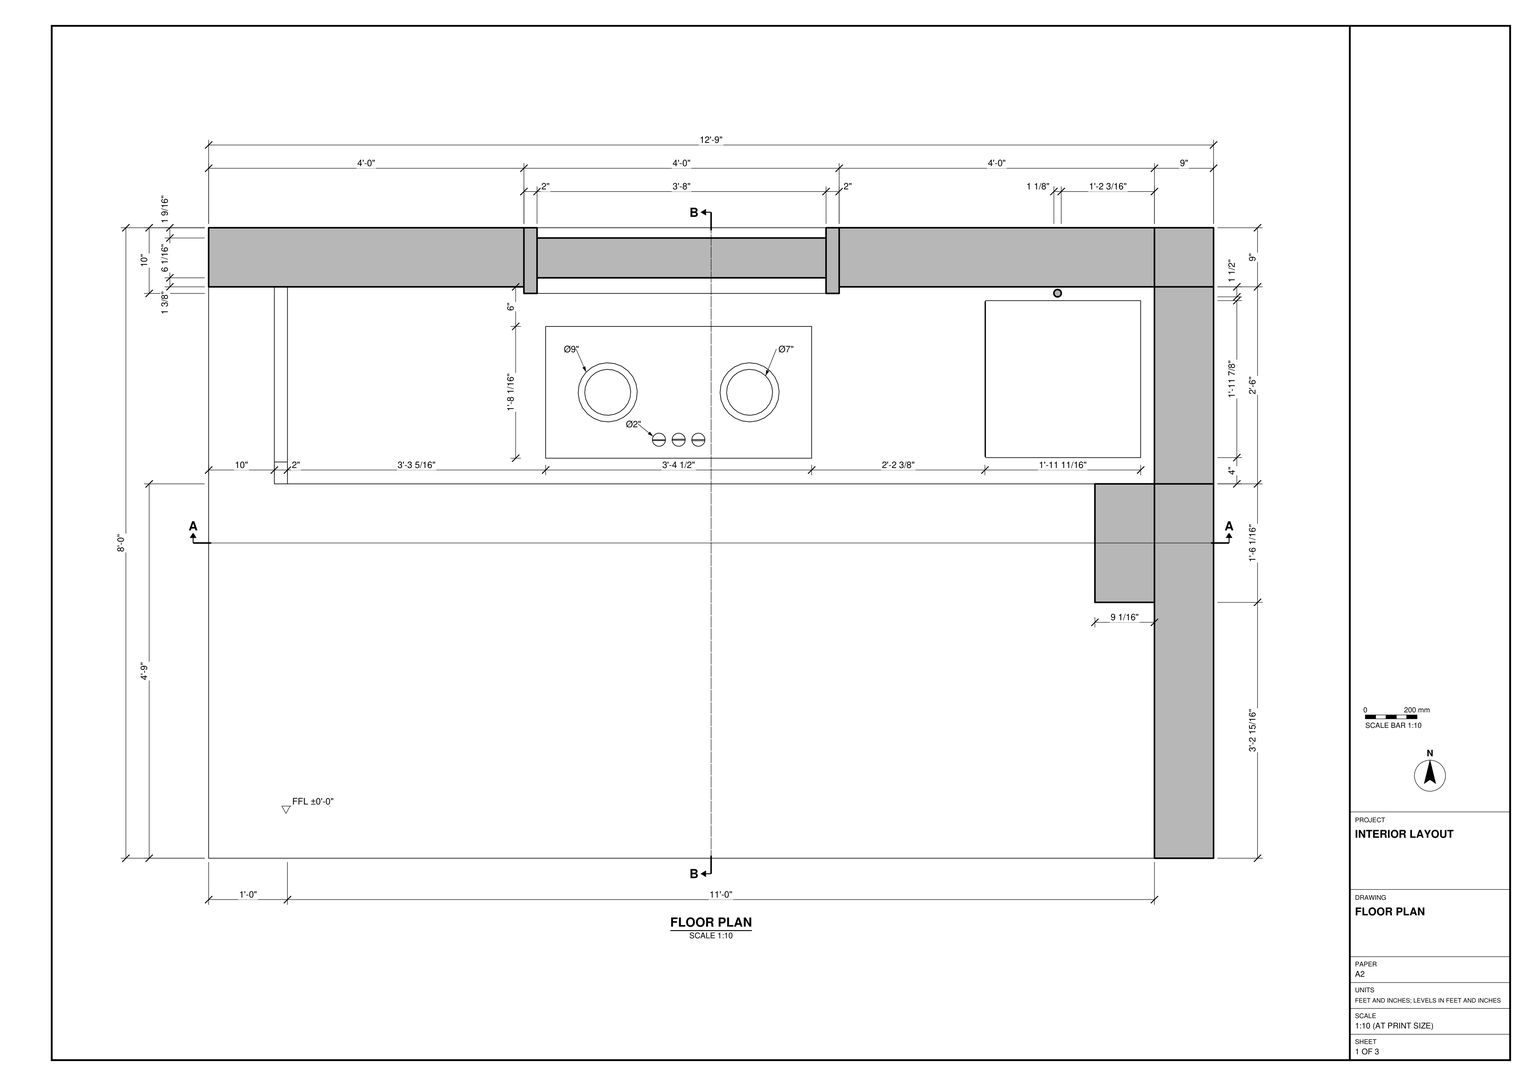
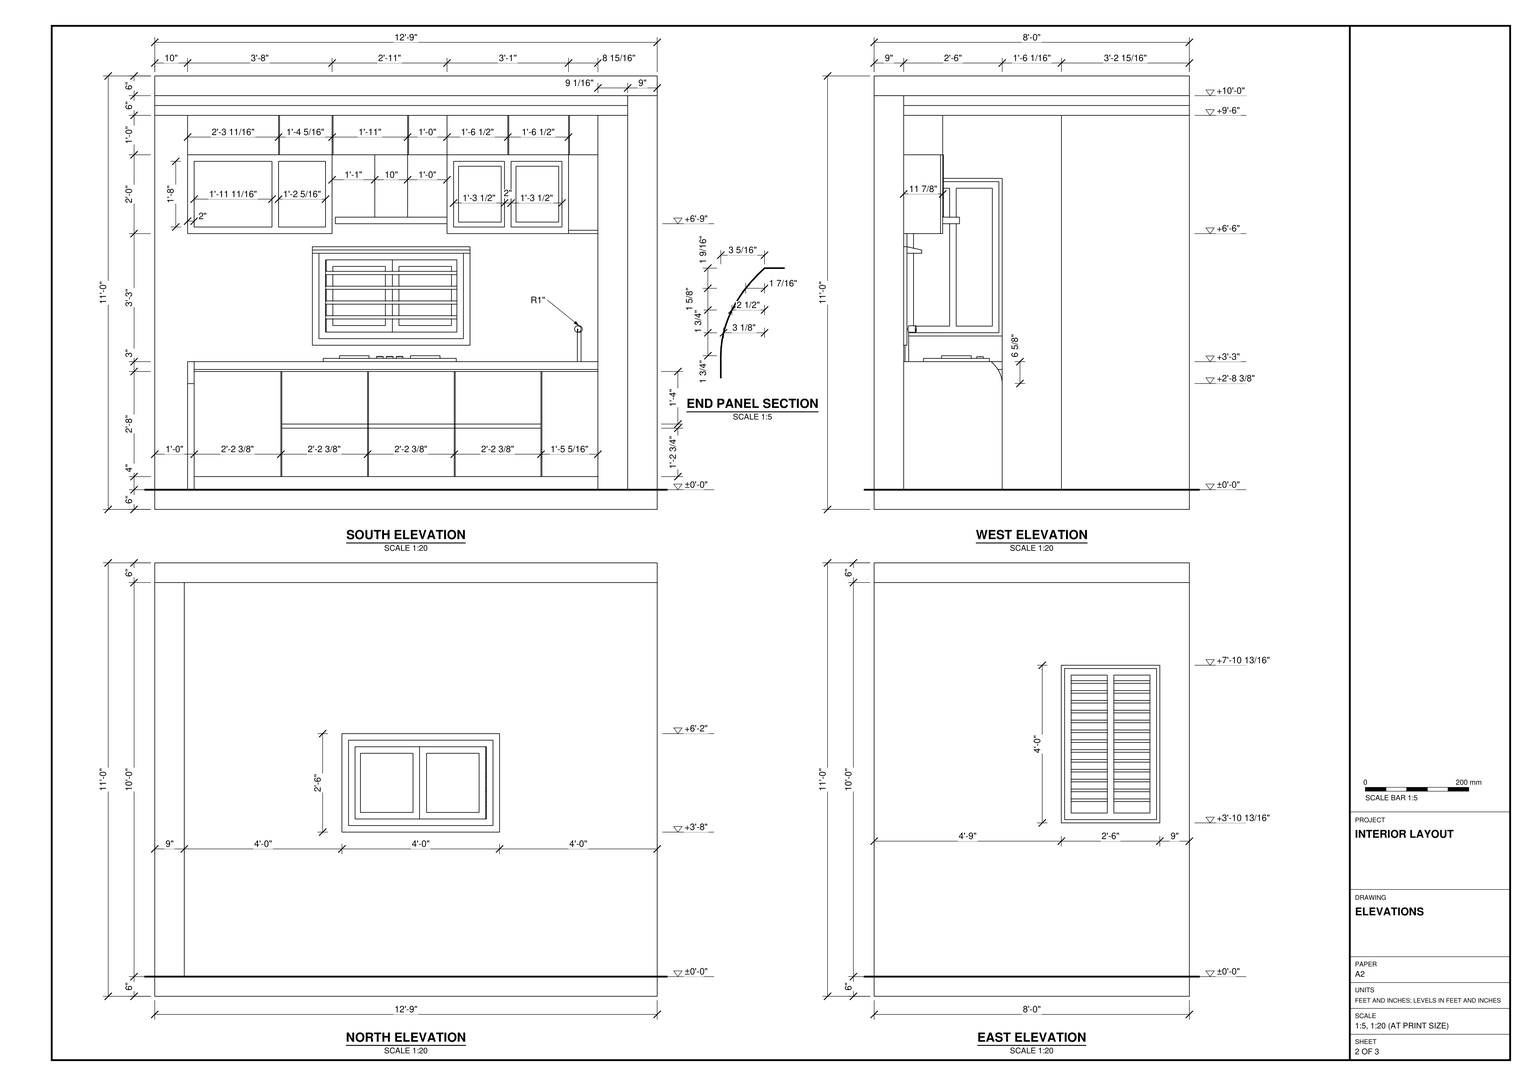
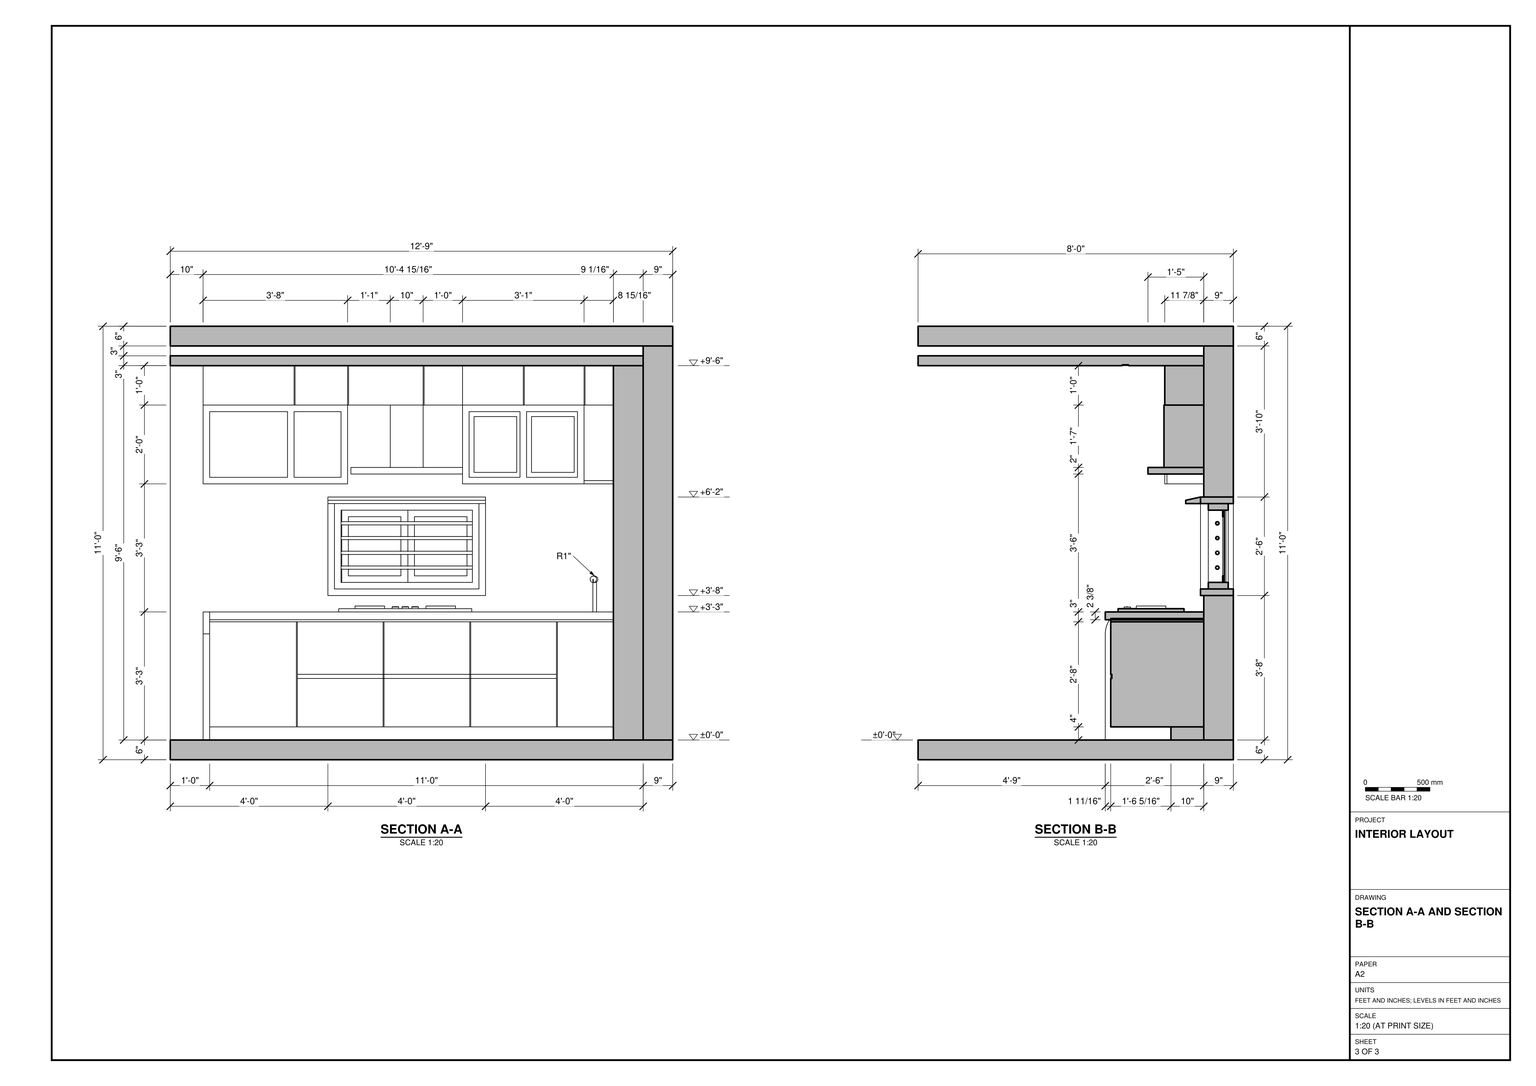
Build the kitchen interior in SketchUp from the plan, elevations and sections in task_files/diagram_01.pdf. Work in feet and inches. The overall model is 12'-9" wide, 8'-0" deep and 11'-0" high, with the finished floor at ±0'-0". Model the floor slab, the 9" thick back and right-hand walls, and the overhead slab. Leave the other two sides open as drawn. Use the sections to set the ceiling below the overhead slab and the elevations to place the two framed windows at their different sill heights.

Build the straight counter run against the back wall. Set the worktop at 3'-3" above the finished floor, with the cooktop beneath the wide window and the sink and tap at the right-hand end. Follow the south elevation for the base cabinet divisions and recessed plinth, and use the end panel section for the curved profile. Match the widths and heights of the upper cabinets and the shelf between the framed cabinet fronts. Decor, appliances and loose items may be any suitable library components.

Keep the walls, slabs, ceiling and each furniture or joinery piece in separate groups or components, and use components for repeated parts. Save one SketchUp model as output_files/kitchen_corner_and_its_built_in_cabinetry.skp.

# SketchUp Ruby script. Lengths in inches.
U = 1.inch
M = Sketchup.active_model
def pt(a) = Geom::Point3d.new(a.map { |v| v * U })
def face(e, loops, mat)
  f = e.add_face(loops[0].map { |a| pt(a) })
  loops[1..].each { |l| e.add_face(l.map { |a| pt(a) }).erase! }
  f.material = f.back_material = mat if mat
  f
end
# faces: each face lists its corners as indices into pts; further lists are holes
def faces(e, pts, list, mat = nil) = list.each { |f| face(e, (f[0].is_a?(Array) ? f : [f]).map { |l| l.map { |i| pts[i] } }, mat) }
# xy, xz, yz: faces in a plane at the given z, y or x. An outline is a flat list of corners, or four numbers for a rectangle; further outlines are holes
def ring(l) = l.size == 4 ? [[l[0], l[1]], [l[2], l[1]], [l[2], l[3]], [l[0], l[3]]] : l.each_slice(2).to_a
def flat(e, list, mat, &to3) = list.each { |f| face(e, (f[0].is_a?(Array) ? f : [f]).map { |l| ring(l).map { |u, v| to3.(u, v) } }, mat) }
def xy(e, z, list, mat = nil) = flat(e, list, mat) { |x, y| [x, y, z] }
def xz(e, y, list, mat = nil) = flat(e, list, mat) { |x, z| [x, y, z] }
def yz(e, x, list, mat = nil) = flat(e, list, mat) { |y, z| [x, y, z] }
def lines(e, pts, list) = list.each { |a, b| e.add_line(pt(pts[a]), pt(pts[b])) }
# prism: a flat outline (further loops are holes) pulled along v
def prism(e, loops, v, mat = nil)
  f = face(e, loops, mat); d = Geom::Vector3d.new(v.map { |x| x * U })
  f.pushpull(f.normal.samedirection?(d) ? d.length : -d.length)
end
def box(e, o, s, mat = nil) = prism(e, [[o, [o[0] + s[0], o[1], o[2]], [o[0] + s[0], o[1] + s[1], o[2]], [o[0], o[1] + s[1], o[2]]]], [0, 0, s[2]], mat)
def at(x, y, z, deg = 0) = Geom::Transformation.translation(pt([x, y, z])) * Geom::Transformation.rotation(ORIGIN, Z_AXIS, deg.degrees)
def axes(o, x, y, z) = Geom::Transformation.new([*x, 0, *y, 0, *z, 0, *pt(o).to_a, 1])
def part(name) = M.definitions.add(name)
# library, detail: a bought-in or finely detailed component or shape, given as its bounding box
def library(name, o, s) = part(name).tap { |d| box(d.entities, o, s) }
def detail(e, o, s) = box(e.add_group.entities, o, s)
def put(e, d, t, mat = nil) = e.add_instance(d, t).tap { |i| i.material = mat if mat }
def group(e, t, mat = nil) = e.add_group.tap { |g| g.transformation = t; g.material = mat if mat }.entities
root = M.entities
M.materials.add("[Color M04]").color = [142, 142, 142]
M.materials.add("[Color M05]").color = [114, 114, 114]
M.materials.add("[Color M06]").color = [86, 86, 86]
M.materials.add("[Color M07]").color = [58, 58, 58]
M.materials.add("[Color M08]").color = [30, 30, 30]
M.materials.add("[Color M09]").color = [0, 0, 0]
M.materials.add("[Concrete Block Layers]").color = [196, 185, 187]
M.materials.add("[Polished Concrete Old]").color = [229, 229, 229]
M.materials.add("[Translucent Glass Gray]").color = [128, 128, 128]
M.materials["[Translucent Glass Gray]"].alpha = 0.5
c1 = library("Group\#21",[0,0,0],[34,17,2])
c2 = part("Group\#34")
prism(c2.entities,[[[0.51,26,0.02],[0.41,26,0],[0.31,26,0.01],[0.21,26,0.05],[0.125,26,0.11],[0.06,26,0.19],[0.02,26,0.28],[0,26,0.39],[0.01,26,0.49],[0.05,26,0.59],[0.11,26,0.67],[0.19,26,0.74],[0.28,26,0.78],[0.39,26,0.8],[0.49,26,0.79],[0.59,26,0.75],[0.67,26,0.69],[0.74,26,0.61],[0.78,26,0.51],[0.8,26,0.41],[0.79,26,0.31],[0.75,26,0.21],[0.69,26,0.125],[0.61,26,0.06]]],[0,-26,0])
c3 = library("Group\#39",[0,0,0],[144,87,3])
c4 = library("Group\#40",[0,0,0],[40.5,20.0625,1.8125])
xz(root,75.45,[[92.5,87.5,105.5,104.5]],"[Translucent Glass Gray]")
xz(root,75.78,[[110,87.5,123,104.5]],"[Translucent Glass Gray]")
g1 = group(root,at(0,60,0))
box(g1,[0,-60,0],[153,96,6])
g2 = group(root,at(48,87,50),"[Concrete Block Layers]")
xy(g2,0,[[0,-1,48,9]])
xy(g2,2,[[2,-1,46,9]])
xy(g2,28,[[2,-1,46,9]])
xy(g2,30,[[0,-1,48,9]])
xz(g2,-1,[[0,0,48,0,48,28,46,28,46,2,2,2,2,28,48,28,48,30,0,30]])
xz(g2,9,[[[0,0,48,30],[2,2,46,28]]])
yz(g2,0,[[-1,0,9,30]])
yz(g2,2,[[-1,2,9,28]])
yz(g2,46,[[-1,2,9,28]])
yz(g2,48,[[-1,0,9,30]])
g3 = group(root,at(50,88.375,52),"[Color M08]")
g4 = group(g3,at(2,2.25,6),"[Color M05]")
prism(g4,[[[0,0.93,0.25],[0,0.85,0.15],[0,0.75,0.07],[0,0.63,0.02],[0,0.5,0],[0,0.37,0.02],[0,0.25,0.07],[0,0.15,0.15],[0,0.07,0.25],[0,0.02,0.37],[0,0,0.5],[0,0.02,0.63],[0,0.07,0.75],[0,0.15,0.85],[0,0.25,0.93],[0,0.37,0.98],[0,0.5,1],[0,0.63,0.98],[0,0.75,0.93],[0,0.85,0.85],[0,0.93,0.75],[0,0.98,0.63],[0,1,0.5],[0,0.98,0.37]]],[40,0,0],"[Color M04]")
yz(g4,0,[[0.5,4.5,0.37,4.52,0.25,4.57,0.15,4.65,0.07,4.75,0.02,4.87,0,5,0.02,5.13,0.07,5.25,0.15,5.35,0.25,5.43,0.37,5.48,0.5,5.5,0.63,5.48,0.75,5.43,0.85,5.35,0.93,5.25,0.98,5.13,1,5,0.98,4.87,0.93,4.75,0.85,4.65,0.75,4.57,0.63,4.52],[0.5,9.02,0.375,9.04,0.26,9.09,0.16,9.16,0.09,9.26,0.04,9.375,0.02,9.5,0.04,9.625,0.09,9.74,0.16,9.84,0.26,9.91,0.375,9.96,0.5,9.98,0.625,9.96,0.74,9.91,0.84,9.84,0.91,9.74,0.96,9.625,0.98,9.5,0.96,9.375,0.91,9.26,0.84,9.16,0.74,9.09,0.625,9.04],[0.47,13.5,0.35,13.52,0.23,13.58,0.13,13.67,0.05,13.77,0.01,13.9,0,14.03,0.02,14.15,0.08,14.27,0.17,14.37,0.27,14.45,0.4,14.49,0.53,14.5,0.65,14.48,0.77,14.42,0.87,14.33,0.95,14.23,0.99,14.1,1,13.97,0.98,13.85,0.92,13.73,0.83,13.63,0.73,13.55,0.6,13.51]])
yz(g4,40,[[0.5,4.5,0.63,4.52,0.75,4.57,0.85,4.65,0.93,4.75,0.98,4.87,1,5,0.98,5.13,0.93,5.25,0.85,5.35,0.75,5.43,0.63,5.48,0.5,5.5,0.37,5.48,0.25,5.43,0.15,5.35,0.07,5.25,0.02,5.13,0,5,0.02,4.87,0.07,4.75,0.15,4.65,0.25,4.57,0.37,4.52],[0.5,9.02,0.625,9.04,0.74,9.09,0.84,9.16,0.91,9.26,0.96,9.375,0.98,9.5,0.96,9.625,0.91,9.74,0.84,9.84,0.74,9.91,0.625,9.96,0.5,9.98,0.375,9.96,0.26,9.91,0.16,9.84,0.09,9.74,0.04,9.625,0.02,9.5,0.04,9.375,0.09,9.26,0.16,9.16,0.26,9.09,0.375,9.04],[0.47,13.5,0.6,13.51,0.73,13.55,0.83,13.63,0.92,13.73,0.98,13.85,1,13.97,0.99,14.1,0.95,14.23,0.87,14.33,0.77,14.42,0.65,14.48,0.53,14.5,0.4,14.49,0.27,14.45,0.17,14.37,0.08,14.27,0.02,14.15,0,14.03,0.01,13.9,0.05,13.77,0.13,13.67,0.23,13.58,0.35,13.52]])
p = [[0,0.25,4.57],[0,0.37,4.52],[40,0.37,4.52],[40,0.25,4.57],[0,0.5,4.5],[40,0.5,4.5],
  [0,0.63,4.52],[40,0.63,4.52],[0,0.75,4.57],[40,0.75,4.57],[0,0.15,4.65],[40,0.15,4.65],
  [0,0.07,4.75],[40,0.07,4.75],[0,0.85,4.65],[40,0.85,4.65],[0,0.93,4.75],[40,0.93,4.75],
  [0,0.02,4.87],[40,0.02,4.87],[0,0.98,4.87],[40,0.98,4.87],[0,0,5],[40,0,5],
  [0,1,5],[40,1,5],[0,0.02,5.13],[40,0.02,5.13],[0,0.98,5.13],[40,0.98,5.13],
  [0,0.07,5.25],[40,0.07,5.25],[0,0.93,5.25],[40,0.93,5.25],[0,0.15,5.35],[40,0.15,5.35],
  [0,0.85,5.35],[40,0.85,5.35],[0,0.25,5.43],[40,0.25,5.43],[0,0.37,5.48],[40,0.37,5.48],
  [0,0.75,5.43],[0,0.63,5.48],[40,0.63,5.48],[40,0.75,5.43],[0,0.5,5.5],[40,0.5,5.5],
  [0,0.26,9.09],[0,0.375,9.04],[40,0.375,9.04],[40,0.26,9.09],[0,0.5,9.02],[40,0.5,9.02],
  [0,0.625,9.04],[40,0.625,9.04],[0,0.74,9.09],[40,0.74,9.09],[0,0.16,9.16],[40,0.16,9.16],
  [0,0.84,9.16],[40,0.84,9.16],[0,0.09,9.26],[40,0.09,9.26],[0,0.91,9.26],[40,0.91,9.26],
  [0,0.04,9.375],[40,0.04,9.375],[0,0.96,9.375],[40,0.96,9.375],[0,0.02,9.5],[40,0.02,9.5],
  [0,0.98,9.5],[40,0.98,9.5],[0,0.04,9.625],[40,0.04,9.625],[0,0.96,9.625],[40,0.96,9.625],
  [0,0.09,9.74],[40,0.09,9.74],[0,0.91,9.74],[40,0.91,9.74],[0,0.16,9.84],[40,0.16,9.84],
  [0,0.84,9.84],[40,0.84,9.84],[0,0.26,9.91],[40,0.26,9.91],[0,0.74,9.91],[40,0.74,9.91],
  [0,0.375,9.96],[40,0.375,9.96],[0,0.625,9.96],[40,0.625,9.96],[0,0.5,9.98],[40,0.5,9.98],
  [0,0.23,13.58],[0,0.35,13.52],[40,0.35,13.52],[40,0.23,13.58],[0,0.47,13.5],[40,0.47,13.5],
  [0,0.6,13.51],[40,0.6,13.51],[0,0.73,13.55],[40,0.73,13.55],[0,0.13,13.67],[40,0.13,13.67],
  [0,0.83,13.63],[40,0.83,13.63],[0,0.92,13.73],[40,0.92,13.73],[0,0.05,13.77],[40,0.05,13.77],
  [0,0.98,13.85],[40,0.98,13.85],[0,0.01,13.9],[40,0.01,13.9],[0,1,13.97],[40,1,13.97],
  [0,0,14.03],[40,0,14.03],[0,0.02,14.15],[40,0.02,14.15],[0,0.99,14.1],[40,0.99,14.1],
  [0,0.95,14.23],[40,0.95,14.23],[0,0.08,14.27],[40,0.08,14.27],[0,0.87,14.33],[40,0.87,14.33],
  [0,0.17,14.37],[40,0.17,14.37],[0,0.77,14.42],[40,0.77,14.42],[0,0.27,14.45],[40,0.27,14.45],
  [0,0.4,14.49],[40,0.4,14.49],[0,0.65,14.48],[40,0.65,14.48],[0,0.53,14.5],[40,0.53,14.5]]
faces(g4,p,[[0,1,2,3],[1,4,5,2],[4,6,7,5],[6,8,9,7],[10,0,3,11],[12,10,11,13],[8,14,15,9],[14,16,17,15],
  [18,12,13,19],[16,20,21,17],[22,18,19,23],[20,24,25,21],[26,22,23,27],[24,28,29,25],[30,26,27,31],[28,32,33,29],
  [34,30,31,35],[32,36,37,33],[38,34,35,39],[40,38,39,41],[42,43,44,45],[36,42,45,37],[46,40,41,47],[43,46,47,44],
  [48,49,50,51],[49,52,53,50],[52,54,55,53],[54,56,57,55],[58,48,51,59],[56,60,61,57],[62,58,59,63],[60,64,65,61],
  [66,62,63,67],[64,68,69,65],[70,66,67,71],[68,72,73,69],[74,70,71,75],[72,76,77,73],[78,74,75,79],[76,80,81,77],
  [82,78,79,83],[80,84,85,81],[86,82,83,87],[84,88,89,85],[90,86,87,91],[88,92,93,89],[94,90,91,95],[92,94,95,93],
  [96,97,98,99],[97,100,101,98],[100,102,103,101],[102,104,105,103],[106,96,99,107],[104,108,109,105],[108,110,111,109],[112,106,107,113],
  [110,114,115,111],[116,112,113,117],[114,118,119,115],[120,116,117,121],[122,120,121,123],[118,124,125,119],[124,126,127,125],[128,122,123,129],
  [126,130,131,127],[132,128,129,133],[130,134,135,131],[136,132,133,137],[138,136,137,139],[134,140,141,135],[142,138,139,143],[140,142,143,141]],"[Color M04]")
g5 = group(g3,at(0,0,0),"[Color M06]")
prism(g5,[[[0,0,26],[0,0,0],[44,0,0],[44,0,26]],[[42,0,2],[2,0,2],[2,0,24],[42,0,24]]],[0,6.0625,0])
g6 = group(g3,at(22.36,4.37,2))
xy(g6,0,[[0,0,20,0.5]])
xy(g6,2,[[2,0,18,0.5]])
xy(g6,20,[[2,0,18,0.5]])
xy(g6,22,[[0,0,20,0.5]])
xz(g6,0,[[[0,0,20,22],[2,2,18,20]]],"[Color M08]")
xz(g6,0.5,[[[0,0,20,22],[2,2,18,20]]])
xz(g6,0.5,[[2,2,18,20]],"[Translucent Glass Gray]")
yz(g6,0,[[0,0,0.5,22]])
yz(g6,2,[[0,2,0.5,20]])
yz(g6,18,[[0,2,0.5,20]])
yz(g6,20,[[0,0,0.5,22]])
g7 = group(g3,at(2.23,4.87,2))
xy(g7,0,[[0,0,20.125,0.5]])
xy(g7,2,[[2,0,18,0.5]])
xy(g7,20,[[2,0,18,0.5]])
xy(g7,22,[[0,0,20.125,0.5]])
xz(g7,0,[[[0,0,20.125,22],[2,2,18,20]]],"[Color M08]")
xz(g7,0.5,[[[0,0,20.125,22],[2,2,18,20]]])
xz(g7,0.5,[[2,2,18,20]],"[Translucent Glass Gray]")
yz(g7,0,[[0,0,0.5,22]])
yz(g7,2,[[0,2,0.5,20]])
yz(g7,18,[[0,2,0.5,20]])
yz(g7,20.125,[[0,0,0.5,22]])
g8 = group(root,at(48,81.5,78),"[Concrete Block Layers]")
prism(g8,[[[0,4.5,2],[0,4.5,0],[0,0,0],[0,0,1]]],[48,0,0])
g9 = group(root,at(10,57,6),"[Polished Concrete Old]")
prism(g9,[[[0,30,39],[0,30,36.95],[0,30,0],[0,0,0],[0,0,32.33],[0,0.02,32.92],[0,0.1,33.51],[0,0.21,34.09],[0,0.38,34.67],[0,0.59,35.25],[0,0.85,35.82],[0,1.16,36.38],[0,1.51,36.93],[0,1.9,37.47],[0,2.34,37.99],[0,2.8125,38.5],[0,3.33,39]]],[2,0,0])
g10 = group(root,at(12,77,6),"[Color M09]")
box(g10,[0,0,0],[132,10,4])
g11 = group(root,at(12,58.67,10))
xy(g11,0,[[0,0,26.4,28.33],[26.7,0,52.8,28.33],[53.1,0,79.2,28.33],[79.5,0,105.6,28.33],[105.9,0,132,28.33],
  [26.4,0.5,26.7,28.33],[52.8,0.5,53.1,28.33],[79.2,0.5,79.5,28.33],[105.6,0.5,105.9,28.33]])
xy(g11,14.74,[[26.7,0,52.8,0.33],[52.8,0,53.1,0.33],[53.1,0,79.2,0.33],[79.2,0,79.5,0.33],[79.5,0,105.6,0.33]])
xy(g11,16,[[26.7,0,52.8,0.33],[52.8,0,53.1,0.33],[53.1,0,79.2,0.33],[79.2,0,79.5,0.33],[79.5,0,105.6,0.33]])
xy(g11,32,[[0,0,26.4,28.33],[26.7,0,52.8,28.33],[53.1,0,79.2,28.33],[79.5,0,105.6,28.33],[105.9,0,132,28.33],
  [26.4,0.5,26.7,28.33],[52.8,0.5,53.1,28.33],[79.2,0.5,79.5,28.33],[105.6,0.5,105.9,28.33]])
xz(g11,0,[[0,0,26.4,32],[26.7,0,52.8,14.74],[53.1,0,79.2,14.74],[79.5,0,105.6,14.74],[105.9,0,132,32],
  [26.7,16,52.8,32],[53.1,16,79.2,32],[79.5,16,105.6,32]])
xz(g11,0.33,[[26.7,14.74,105.6,16]],"[Color M09]")
xz(g11,0.5,[[26.4,0,26.7,32],[52.8,0,53.1,32],[79.2,0,79.5,32],[105.6,0,105.9,32]])
xz(g11,28.33,[[0,0,26.4,32],[26.4,0,26.7,32],[26.7,0,52.8,32],[52.8,0,53.1,32],[53.1,0,79.2,32],
  [79.2,0,79.5,32],[79.5,0,105.6,32],[105.6,0,105.9,32],[105.9,0,132,32]])
yz(g11,0,[[0,0,28.33,32]])
yz(g11,26.4,[[0,0,0.5,32],[0.5,0,28.33,32]])
yz(g11,26.7,[[0,0,0.5,0,0.5,32,0,32,0,16,0.33,16,0.33,14.74,0,14.74],[0.5,0,28.33,32]])
yz(g11,52.8,[[0.5,0,28.33,32]])
yz(g11,53.1,[[0.5,0,28.33,32]])
yz(g11,79.2,[[0.5,0,28.33,32]])
yz(g11,79.5,[[0.5,0,28.33,32]])
yz(g11,105.6,[[0,0,0.5,0,0.5,32,0,32,0,16,0.33,16,0.33,14.74,0,14.74],[0.5,0,28.33,32]])
yz(g11,105.9,[[0,0,0.5,32],[0.5,0,28.33,32]])
yz(g11,132,[[0,0,28.33,32]])
g12 = group(root,at(12,60.33,42),"[Color M09]")
g13 = group(g12,at(0,0,0))
xy(g13,-1.5,[[106.19,0.67,130,24.67]])
xy(g13,0,[[0,-1.67,132,26.67]])
xy(g13,1,[[[0,-1.67,132,26.67],[106.19,0.67,130,24.67]]])
xz(g13,-1.67,[[0,0,132,1]])
xz(g13,0.67,[[106.19,-1.5,130,1]])
xz(g13,24.67,[[106.19,-1.5,130,1]])
xz(g13,26.67,[[0,0,132,1]])
yz(g13,0,[[-1.67,0,26.67,1]])
yz(g13,106.19,[[0.67,-1.5,24.67,1]])
yz(g13,130,[[0.67,-1.5,24.67,1]])
yz(g13,132,[[-1.67,0,26.67,1]])
g14 = group(root,at(12,58.67,43),"[Polished Concrete Old]")
xy(g14,-0.6875,[[106.29,2.33,129.9,26.23]],"[Color M07]")
xy(g14,-0.375,[[0,-1.67,132,28.33]],"[Color M09]")
xy(g14,2,[[[0,-1.67,132,28.33],[106.29,2.33,129.9,26.23]]])
xz(g14,-1.67,[[0,-0.375,132,2]])
xz(g14,2.33,[[106.29,-0.6875,129.9,2]])
xz(g14,26.23,[[106.29,-0.6875,129.9,2]],"[Color M07]")
xz(g14,28.33,[[0,-0.375,132,2]])
yz(g14,0,[[-1.67,-0.375,28.33,2]])
yz(g14,106.29,[[2.33,-0.6875,26.23,2]],"[Color M07]")
yz(g14,129.9,[[2.33,-0.6875,26.23,2]],"[Color M07]")
yz(g14,132,[[-1.67,-0.375,28.33,2]])
g15 = group(root,at(12,70,94.5))
box(g15,[0,5.75,0],[23.7,11.25,1.5])
g16 = group(root,at(37.7,70,94.5))
box(g16,[0,5.81,0],[14.3,11.19,1.5])
g17 = group(root,at(10,75.12,84))
g18 = group(g17,at(0,0.66,0))
xy(g18,0,[[0,0,44,11.22]])
xy(g18,0,[[0,-0.66,44,0]],"[Color M09]")
xy(g18,2,[[2,-0.66,25.7,0],[27.7,-0.66,42,0],[2,0,25.7,11.22],[27.7,0,42,11.22]])
xy(g18,22,[[2,-0.66,25.7,0],[27.7,-0.66,42,0],[2,0,25.7,11.22],[27.7,0,42,11.22]])
xy(g18,24,[[0,0,44,11.22]])
xy(g18,24,[[0,-0.66,44,0]],"[Color M09]")
xz(g18,-0.66,[[[0,0,44,24],[2,2,25.7,22],[27.7,2,42,22]]],"[Color M09]")
xz(g18,0,[[[0,0,44,24],[2,2,25.7,22],[27.7,2,42,22]]])
xz(g18,11.22,[[[0,0,44,24],[2,2,25.7,22],[27.7,2,42,22]]])
yz(g18,0,[[0,0,11.22,24]])
yz(g18,0,[[-0.66,0,0,24]],"[Color M09]")
yz(g18,2,[[-0.66,2,0,22],[0,2,11.22,22]])
yz(g18,25.7,[[-0.66,2,0,22],[0,2,11.22,22]])
yz(g18,27.7,[[-0.66,2,0,22],[0,2,11.22,22]])
yz(g18,42,[[-0.66,2,0,22],[0,2,11.22,22]])
yz(g18,44,[[0,0,11.22,24]])
yz(g18,44,[[-0.66,0,0,24]],"[Color M09]")
g19 = group(g17,at(2,0,2))
xz(g19,0,[[0,0,23.7,20]],"[Translucent Glass Gray]")
g20 = group(g17,at(27.7,0,2))
xz(g20,0,[[0,0,14.3,20]],"[Translucent Glass Gray]")
put(root,c1,at(55,70,87))
g21 = group(root,at(67,74.875,89),"[Color M09]")
box(g21,[0,0,0],[10,12.125,19])
g22 = group(root,at(89,75.12,84))
xy(g22,0,[[0,0.66,37,11.88]])
xy(g22,0,[[0,0,37,0.66]],"[Color M08]")
xy(g22,2,[[2,0,17.5,0.66],[19.5,0,35,0.66],[2,0.66,17.5,11.88],[19.5,0.66,35,11.88]])
xy(g22,22,[[2,0,17.5,0.66],[19.5,0,35,0.66],[2,0.66,17.5,11.88],[19.5,0.66,35,11.88]])
xy(g22,24,[[0,0.66,37,11.88]])
xy(g22,24,[[0,0,37,0.66]],"[Color M08]")
xz(g22,0,[[[0,0,37,24],[2,2,17.5,22],[19.5,2,35,22]]],"[Color M08]")
xz(g22,0.66,[[[0,0,37,24],[2,2,17.5,22],[19.5,2,35,22]]])
xz(g22,11.88,[[[0,0,37,24],[2,2,17.5,22],[19.5,2,35,22]]])
yz(g22,0,[[0.66,0,11.88,24]])
yz(g22,0,[[0,0,0.66,24]],"[Color M08]")
yz(g22,2,[[0,2,0.66,22],[0.66,2,11.88,22]])
yz(g22,17.5,[[0,2,0.66,22],[0.66,2,11.88,22]])
yz(g22,19.5,[[0,2,0.66,22],[0.66,2,11.88,22]])
yz(g22,35,[[0,2,0.66,22],[0.66,2,11.88,22]])
yz(g22,37,[[0,0,0.66,24],[0.66,0,11.88,24]])
g23 = group(root,at(91,75.45,86))
prism(g23,[[[0,0,20],[0,0,0],[15.5,0,0],[15.5,0,20]],[[14.5,0,1.5],[1.5,0,1.5],[1.5,0,18.5],[14.5,0,18.5]]],[0,1,0],"[Color M07]")
g24 = group(root,at(108.5,75.78,86))
prism(g24,[[[0,0,20],[0,0,0],[15.5,0,0],[15.5,0,20]],[[14.5,0,1.5],[1.5,0,1.5],[1.5,0,18.5],[14.5,0,18.5]]],[0,1,0],"[Color M07]")
g25 = group(root,at(0,87,6))
prism(g25,[[[0,0,0],[144,0,0],[144,0,120],[0,0,120]],[[96,0,74],[96,0,44],[48,0,44],[48,0,74]]],[0,9,0])
g26 = group(root,at(91,76.45,96))
box(g26,[0,0,0],[15.5,10.55,1])
g27 = group(root,at(108.5,76.78,96))
box(g27,[0,0,0],[15.5,10.22,1])
g28 = group(root,at(126,75.12,84))
xy(g28,0,[[0,0,8.9375,11.88]],"[Color M09]")
xy(g28,1,[[0,0,8.9375,11.88]])
xy(g28,24,[[0,0,8.9375,11.88]])
xz(g28,0,[[0,1,8.9375,24]])
xz(g28,0,[[0,0,8.9375,1]],"[Color M09]")
xz(g28,11.88,[[0,0,8.9375,1],[0,1,8.9375,24]])
yz(g28,0,[[0,0,11.88,1],[0,1,11.88,24]])
yz(g28,8.9375,[[0,0,11.88,1],[0,1,11.88,24]])
g29 = group(root,at(10,75.12,108))
xy(g29,0,[[0,0,27.7,11.88],[27.7,0,28,11.88],[28,0,44,11.88],[44,0,44.3,11.88],[44.3,0,67,11.88],
  [67,0,67.3,11.88],[67.3,0,79,11.88],[79,0,97.5,11.88],[97.5,0,97.8,11.88],[97.8,0,116,11.88],
  [116,0,116.3,11.88],[116.3,0,124.9375,11.88]])
xy(g29,12,[[0,0,27.7,11.88],[27.7,0,28,11.88],[28,0,44,11.88],[44,0,44.3,11.88],[44.3,0,67,11.88],
  [67,0,67.3,11.88],[67.3,0,79,11.88],[79,0,97.5,11.88],[97.5,0,97.8,11.88],[97.8,0,116,11.88],
  [116,0,116.3,11.88],[116.3,0,124.9375,11.88]])
xz(g29,0,[[0,0,27.7,12],[27.7,0,28,12],[28,0,44,12],[44,0,44.3,12],[44.3,0,67,12],
  [67,0,67.3,12],[67.3,0,79,12],[79,0,97.5,12],[97.5,0,97.8,12],[97.8,0,116,12],
  [116,0,116.3,12],[116.3,0,124.9375,12]])
xz(g29,11.88,[[0,0,27.7,12],[27.7,0,28,12],[28,0,44,12],[44,0,44.3,12],[44.3,0,67,12],
  [67,0,67.3,12],[67.3,0,79,12],[79,0,97.5,12],[97.5,0,97.8,12],[97.8,0,116,12],
  [116,0,116.3,12],[116.3,0,124.9375,12]])
yz(g29,0,[[0,0,11.88,12]])
yz(g29,27.7,[[0,0,11.88,12]])
yz(g29,28,[[0,0,11.88,12]])
yz(g29,44,[[0,0,11.88,12]])
yz(g29,44.3,[[0,0,11.88,12]])
yz(g29,67,[[0,0,11.88,12]])
yz(g29,67.3,[[0,0,11.88,12]])
yz(g29,79,[[0,0,11.88,12]])
yz(g29,97.5,[[0,0,11.88,12]])
yz(g29,97.8,[[0,0,11.88,12]])
yz(g29,116,[[0,0,11.88,12]])
yz(g29,116.3,[[0,0,11.88,12]])
yz(g29,124.9375,[[0,0,11.88,12]])
g30 = group(root,at(144,0,6))
prism(g30,[[[9,0,0],[9,96,0],[9,96,120],[9,0,120]],[[9,57,94.8125],[9,87,94.8125],[9,87,46.8125],[9,57,46.8125]]],[-9,0,0])
g31 = group(root,at(134.9375,38.96,6))
prism(g31,[[[0,0,114],[0,48.04,114],[0,48.04,94.8125],[0,18.04,94.8125],[0,18.04,0],[0,0,0]]],[9.0625,0,0])
g32 = group(root,at(144,57,52.8125),"[Concrete Block Layers]")
g33 = group(g32,at(0,0,0))
yz(g33,2.5625,[[3,3,14,45],[16,3,27,45]],"[Translucent Glass Gray]")
g34 = group(g33,at(0,0,0))
prism(g34,[[[9,30,0],[9,30,48],[9,0,48],[9,0,0]],[[9,1,47],[9,29,47],[9,29,1],[9,1,1]]],[-9,0,0])
g35 = group(g33,at(2.5625,1,1),"[Color M09]")
prism(g35,[[[0,28,0],[0,0,0],[0,0,46],[0,28,46]],[[0,13,2],[0,13,44],[0,2,44],[0,2,2]],[[0,26,44],[0,15,44],[0,15,2],[0,26,2]]],[3,0,0])
g36 = group(g32,at(3.66,1,6.5),"[Color M06]")
put(g36,c2,at(0,0,0))
put(g36,c2,at(0,0,27))
put(g36,c2,at(0,0,36))
put(g36,c2,at(0,0,24))
put(g36,c2,at(0,0,9))
put(g36,c2,at(0,0,33))
put(g36,c2,at(0,0,30))
put(g36,c2,at(0,0,3))
put(g36,c2,at(0,0,6))
put(g36,c2,at(0,0,15))
put(g36,c2,at(0,0,21))
put(g36,c2,at(0,0,18))
put(g36,c2,at(0,0,12))
put(root,c3,at(0,0,120))
put(root,c4,at(51.31,60.91,45),"[Color M08]")
g37 = group(root,at(127.85,83.14,45))
xy(g37,0,[[1.375,2.33,1.23,2.36,1.1,2.42,0.99,2.52,0.9,2.64,0.85,2.77,0.84,2.92,0.87,3.07,0.93,3.2,1.03,3.31,1.15,3.39,1.28,3.44,1.43,3.45,1.58,3.43,1.71,3.37,1.82,3.27,1.9,3.15,1.95,3.01,1.96,2.87,1.9375,2.72,1.875,2.59,1.78,2.48,1.66,2.39,1.52,2.34]])
xy(g37,9.9375,[[0.98,0.18,0.84,0.21,1.23,2.36,1.375,2.33],[1.375,2.33,1.52,2.34,1.66,2.39,1.78,2.48,1.875,2.59,1.9375,2.72,1.96,2.87,1.95,3.01,1.9,3.15,1.82,3.27,1.71,3.37,1.58,3.43,1.43,3.45,1.28,3.44,1.15,3.39,1.03,3.31,0.93,3.2,0.87,3.07,0.84,2.92,0.85,2.77,0.9,2.64,0.99,2.52,1.1,2.42,1.23,2.36]])
p = [[1.375,2.33,0],[1.375,2.33,8.9375],[1.23,2.36,8.96],[1.23,2.36,0],[1.52,2.34,0],[1.52,2.34,9.9375],
  [1.375,2.33,9.9375],[1.66,2.39,0],[1.66,2.39,9.9375],[0.99,2.52,0],[1.1,2.42,0],[1.1,2.42,9.9375],
  [0.99,2.52,9.9375],[1.23,2.36,9.9375],[1.78,2.48,0],[1.78,2.48,9.9375],[0.9,2.64,0],[0.9,2.64,9.9375],
  [1.875,2.59,0],[1.875,2.59,9.9375],[0.85,2.77,0],[0.85,2.77,9.9375],[1.9375,2.72,0],[1.9375,2.72,9.9375],
  [1.96,2.87,0],[1.96,2.87,9.9375],[0.84,2.92,0],[0.84,2.92,9.9375],[0.87,3.07,0],[0.87,3.07,9.9375],
  [1.95,3.01,0],[1.95,3.01,9.9375],[1.9,3.15,0],[1.9,3.15,9.9375],[0.93,3.2,0],[0.93,3.2,9.9375],
  [1.03,3.31,0],[1.03,3.31,9.9375],[1.82,3.27,0],[1.82,3.27,9.9375],[1.15,3.39,0],[1.15,3.39,9.9375],
  [1.71,3.37,0],[1.71,3.37,9.9375],[1.28,3.44,0],[1.28,3.44,9.9375],[1.43,3.45,0],[1.43,3.45,9.9375],
  [1.58,3.43,0],[1.58,3.43,9.9375],[0.98,0.18,8.9375],[1.24,0.13,8.97],[1.48,0.09,9.07],[1.68,0.05,9.23],
  [1.84,0.02,9.4375],[1.93,0.01,9.68],[1.97,0,9.9375],[1.93,0.01,10.2],[1.84,0.02,10.4375],[1.68,0.05,10.64],
  [1.48,0.09,10.8],[1.24,0.13,10.9],[0.98,0.18,10.9375],[0.73,0.23,10.9],[0.49,0.27,10.8],[0.29,0.31,10.64],
  [0.13,0.33,10.4375],[0.03,0.35,10.2],[0,0.36,9.9375],[0.03,0.35,9.68],[0.13,0.33,9.4375],[0.29,0.31,9.23],
  [0.49,0.27,9.07],[0.73,0.23,8.97],[0.84,0.21,8.96],[0.84,0.21,9.9375],[0.98,0.18,9.9375],[1.63,2.28,8.97],
  [1.12,2.38,8.97],[0.88,2.42,9.07],[0.68,2.46,9.23],[0.52,2.49,9.4375],[0.43,2.5,9.68],[0.39,2.51,9.9375],
  [0.43,2.5,10.2],[0.52,2.49,10.4375],[0.68,2.46,10.64],[0.88,2.42,10.8],[1.12,2.38,10.9],[1.375,2.33,10.9375],
  [1.63,2.28,10.9],[1.87,2.24,10.8],[2.07,2.2,10.64],[2.23,2.18,10.4375],[2.33,2.16,10.2],[2.36,2.15,9.9375],
  [2.33,2.16,9.68],[2.23,2.18,9.4375],[2.07,2.2,9.23],[1.87,2.24,9.07]]
faces(g37,p,[[0,1,2,3],[0,4,5,6,1],[4,7,8,5],[9,10,11,12],[10,3,2,13,11],[7,14,15,8],[16,9,12,17],[14,18,19,15],
  [20,16,17,21],[18,22,23,19],[22,24,25,23],[26,20,21,27],[28,26,27,29],[24,30,31,25],[30,32,33,31],[34,28,29,35],
  [36,34,35,37],[32,38,39,33],[40,36,37,41],[38,42,43,39],[44,40,41,45],[46,44,45,47],[48,46,47,49],[42,48,49,43],
  [50,51,52,53,54,55,56,57,58,59,60,61,62,63,64,65,66,67,68,69,70,71,72,73,74,75,76],[1,77,51,50],[77,99,52,51],[79,78,73,72],[78,2,74,73],[99,98,53,52],[80,79,72,71],[98,97,54,53],
  [81,80,71,70],[97,96,55,54],[82,81,70,69],[96,95,56,55],[83,82,69,68],[95,94,57,56],[84,83,68,67],[94,93,58,57],
  [85,84,67,66],[93,92,59,58],[86,85,66,65],[92,91,60,59],[87,86,65,64],[91,90,61,60],[88,87,64,63],[90,89,62,61],
  [89,88,63,62]],"[Color M07]")
faces(g37,p,[[6,1,50,76],[77,1,6,13,2,78,79,80,81,82,83,84,85,86,87,88,89,90,91,92,93,94,95,96,97,98,99],[13,2,1,6],[2,13,75,74]])
g38 = group(root,at(0,0,126))
box(g38,[0,0,0],[153,96,6])
